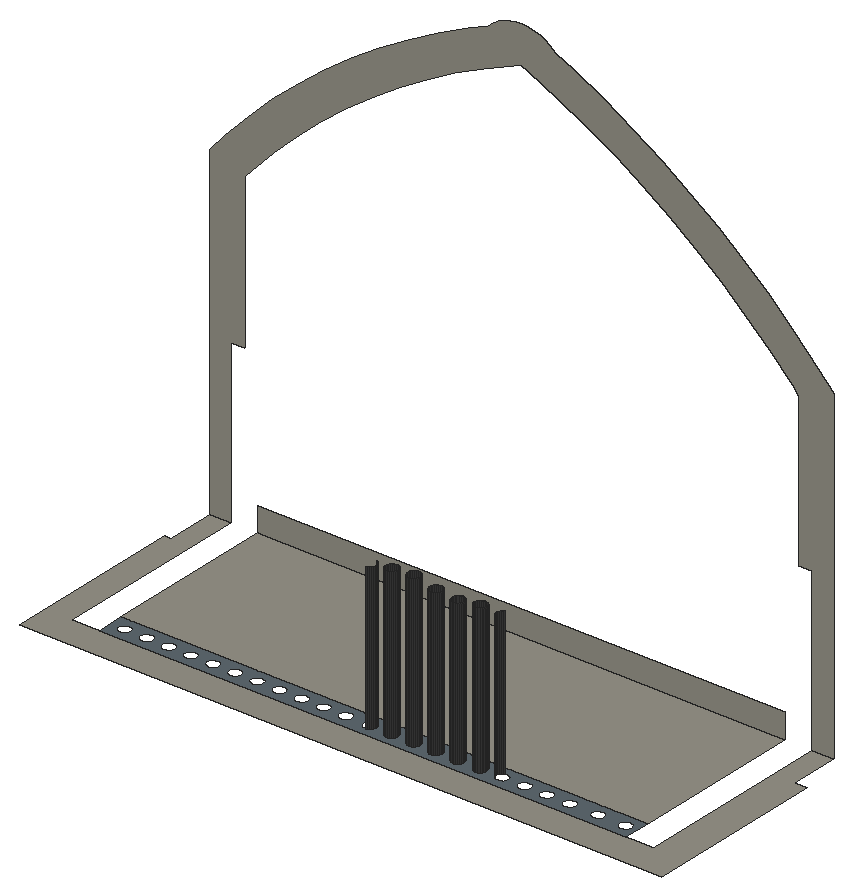
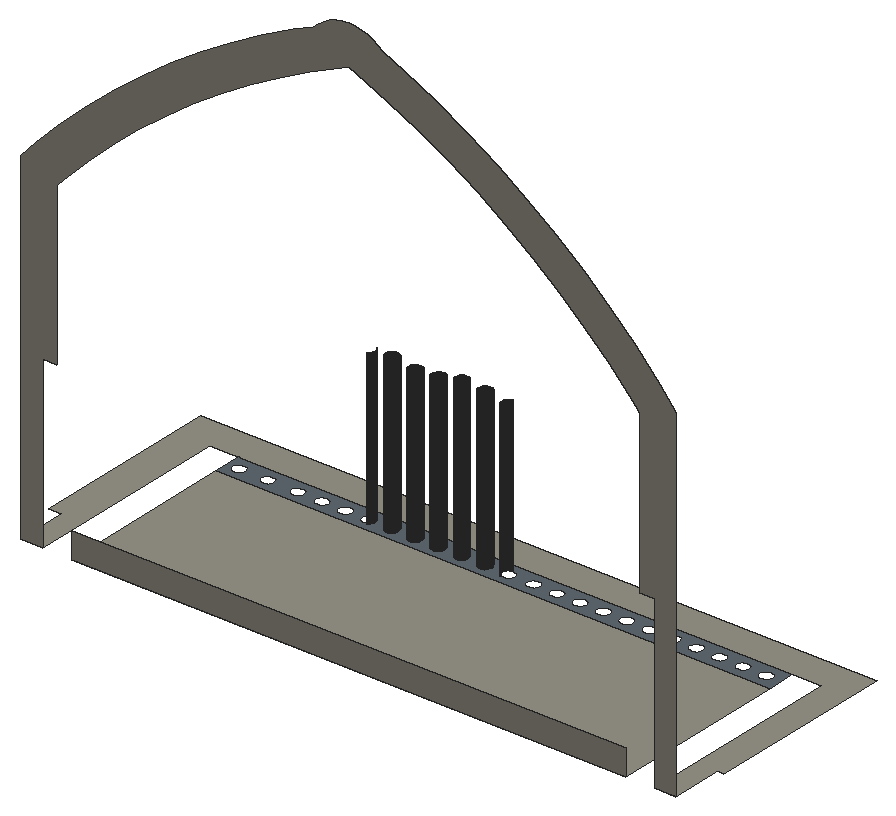
# SketchUp Ruby script. Lengths in inches.
U = 1.inch
M = Sketchup.active_model
def pt(a) = Geom::Point3d.new(a.map { |v| v * U })
def face(e, loops, mat)
  f = e.add_face(loops[0].map { |a| pt(a) })
  loops[1..].each { |l| e.add_face(l.map { |a| pt(a) }).erase! }
  f.material = f.back_material = mat if mat
  f
end
# faces: each face lists its corners as indices into pts; further lists are holes
def faces(e, pts, list, mat = nil) = list.each { |f| face(e, (f[0].is_a?(Array) ? f : [f]).map { |l| l.map { |i| pts[i] } }, mat) }
# xy, xz, yz: faces in a plane at the given z, y or x. An outline is a flat list of corners, or four numbers for a rectangle; further outlines are holes
def ring(l) = l.size == 4 ? [[l[0], l[1]], [l[2], l[1]], [l[2], l[3]], [l[0], l[3]]] : l.each_slice(2).to_a
def flat(e, list, mat, &to3) = list.each { |f| face(e, (f[0].is_a?(Array) ? f : [f]).map { |l| ring(l).map { |u, v| to3.(u, v) } }, mat) }
def xy(e, z, list, mat = nil) = flat(e, list, mat) { |x, y| [x, y, z] }
def xz(e, y, list, mat = nil) = flat(e, list, mat) { |x, z| [x, y, z] }
def yz(e, x, list, mat = nil) = flat(e, list, mat) { |y, z| [x, y, z] }
def lines(e, pts, list) = list.each { |a, b| e.add_line(pt(pts[a]), pt(pts[b])) }
# prism: a flat outline (further loops are holes) pulled along v
def prism(e, loops, v, mat = nil)
  f = face(e, loops, mat); d = Geom::Vector3d.new(v.map { |x| x * U })
  f.pushpull(f.normal.samedirection?(d) ? d.length : -d.length)
end
def box(e, o, s, mat = nil) = prism(e, [[o, [o[0] + s[0], o[1], o[2]], [o[0] + s[0], o[1] + s[1], o[2]], [o[0], o[1] + s[1], o[2]]]], [0, 0, s[2]], mat)
def at(x, y, z, deg = 0) = Geom::Transformation.translation(pt([x, y, z])) * Geom::Transformation.rotation(ORIGIN, Z_AXIS, deg.degrees)
def axes(o, x, y, z) = Geom::Transformation.new([*x, 0, *y, 0, *z, 0, *pt(o).to_a, 1])
def part(name) = M.definitions.add(name)
# library, detail: a bought-in or finely detailed component or shape, given as its bounding box
def library(name, o, s) = part(name).tap { |d| box(d.entities, o, s) }
def detail(e, o, s) = box(e.add_group.entities, o, s)
def put(e, d, t, mat = nil) = e.add_instance(d, t).tap { |i| i.material = mat if mat }
def group(e, t, mat = nil) = e.add_group.tap { |g| g.transformation = t; g.material = mat if mat }.entities
root = M.entities
M.materials.add("[Color M07]").color = [58, 58, 58]
M.materials.add("[Formica Graystone]").color = [149, 146, 135]
M.materials.add("[Formica Speckled Grey]").color = [94, 105, 111]
xy(root,452.9,[[260.4,119.22,260.2,119.27,260.01,119.375,259.86,119.52,259.75,119.71,259.69,119.91,259.69,120.125,259.75,120.33,259.85,120.51,260,120.67,260.18,120.77,260.38,120.83,260.6,120.83,260.8,120.78,260.99,120.68,261.14,120.53,261.25,120.35,261.3,120.14,261.31,119.93,261.25,119.72,261.15,119.54,261,119.39,260.82,119.28,260.61,119.22],[263.28,119.22,263.07,119.27,262.89,119.375,262.73,119.52,262.625,119.71,262.57,119.91,262.57,120.125,262.62,120.33,262.72,120.51,262.87,120.67,263.05,120.77,263.26,120.83,263.47,120.83,263.68,120.78,263.86,120.68,264.01,120.53,264.12,120.35,264.18,120.14,264.18,119.93,264.13,119.72,264.02,119.54,263.875,119.39,263.69,119.28,263.49,119.22],[266.15,119.22,265.95,119.27,265.76,119.375,265.61,119.52,265.5,119.71,265.44,119.91,265.44,120.125,265.5,120.33,265.6,120.51,265.75,120.67,265.93,120.77,266.13,120.83,266.35,120.83,266.55,120.78,266.74,120.68,266.89,120.53,267,120.35,267.05,120.14,267.06,119.93,267,119.72,266.9,119.54,266.75,119.39,266.57,119.28,266.36,119.22],[269.03,119.22,268.82,119.27,268.64,119.375,268.48,119.52,268.375,119.71,268.32,119.91,268.32,120.125,268.37,120.33,268.47,120.51,268.62,120.67,268.8,120.77,269.01,120.83,269.22,120.83,269.43,120.78,269.61,120.68,269.76,120.53,269.87,120.35,269.93,120.14,269.93,119.93,269.88,119.72,269.77,119.54,269.625,119.39,269.44,119.28,269.24,119.22],[271.9,119.22,271.7,119.27,271.51,119.375,271.36,119.52,271.25,119.71,271.19,119.91,271.19,120.125,271.25,120.33,271.35,120.51,271.5,120.67,271.68,120.77,271.88,120.83,272.1,120.83,272.3,120.78,272.49,120.68,272.64,120.53,272.75,120.35,272.8,120.14,272.81,119.93,272.75,119.72,272.65,119.54,272.5,119.39,272.32,119.28,272.11,119.22]])
xy(root,452.9,[[216.84,114.16,300.34,114.16,300.34,137.66,298.71,137.66,298.71,144.04,295.93,144.04,295.93,118.22,220.36,118.22,220.36,144.04,217.65,144.04,217.65,137.66,216.84,137.66],[223.91,121.78,292.38,144.04]],"[Formica Graystone]")
xy(root,452.9,[[[223.91,118.22,292.38,121.78],[225.65,119.22,225.45,119.27,225.26,119.375,225.11,119.52,225,119.71,224.94,119.91,224.94,120.125,225,120.33,225.1,120.51,225.25,120.67,225.43,120.77,225.63,120.83,225.85,120.83,226.05,120.78,226.24,120.68,226.39,120.53,226.5,120.35,226.55,120.14,226.56,119.93,226.5,119.72,226.4,119.54,226.25,119.39,226.07,119.28,225.86,119.22],[228.53,119.22,228.32,119.27,228.14,119.375,227.98,119.52,227.875,119.71,227.82,119.91,227.82,120.125,227.87,120.33,227.97,120.51,228.12,120.67,228.3,120.77,228.51,120.83,228.72,120.83,228.93,120.78,229.11,120.68,229.26,120.53,229.37,120.35,229.43,120.14,229.43,119.93,229.38,119.72,229.27,119.54,229.125,119.39,228.94,119.28,228.74,119.22],[231.4,119.22,231.2,119.27,231.01,119.375,230.86,119.52,230.75,119.71,230.69,119.91,230.69,120.125,230.75,120.33,230.85,120.51,231,120.67,231.18,120.77,231.38,120.83,231.6,120.83,231.8,120.78,231.99,120.68,232.14,120.53,232.25,120.35,232.3,120.14,232.31,119.93,232.25,119.72,232.15,119.54,232,119.39,231.82,119.28,231.61,119.22],[234.28,119.22,234.07,119.27,233.89,119.375,233.73,119.52,233.625,119.71,233.57,119.91,233.57,120.125,233.62,120.33,233.72,120.51,233.87,120.67,234.05,120.77,234.26,120.83,234.47,120.83,234.68,120.78,234.86,120.68,235.01,120.53,235.12,120.35,235.18,120.14,235.18,119.93,235.13,119.72,235.02,119.54,234.875,119.39,234.69,119.28,234.49,119.22],[237.15,119.22,236.95,119.27,236.76,119.375,236.61,119.52,236.5,119.71,236.44,119.91,236.44,120.125,236.5,120.33,236.6,120.51,236.75,120.67,236.93,120.77,237.13,120.83,237.35,120.83,237.55,120.78,237.74,120.68,237.89,120.53,238,120.35,238.05,120.14,238.06,119.93,238,119.72,237.9,119.54,237.75,119.39,237.57,119.28,237.36,119.22],[240.03,119.22,239.82,119.27,239.64,119.375,239.48,119.52,239.375,119.71,239.32,119.91,239.32,120.125,239.37,120.33,239.47,120.51,239.62,120.67,239.8,120.77,240.01,120.83,240.22,120.83,240.43,120.78,240.61,120.68,240.76,120.53,240.87,120.35,240.93,120.14,240.93,119.93,240.88,119.72,240.77,119.54,240.625,119.39,240.44,119.28,240.24,119.22],[242.9,119.22,242.7,119.27,242.51,119.375,242.36,119.52,242.25,119.71,242.19,119.91,242.19,120.125,242.25,120.33,242.35,120.51,242.5,120.67,242.68,120.77,242.88,120.83,243.1,120.83,243.3,120.78,243.49,120.68,243.64,120.53,243.75,120.35,243.8,120.14,243.81,119.93,243.75,119.72,243.65,119.54,243.5,119.39,243.32,119.28,243.11,119.22],[245.78,119.22,245.57,119.27,245.39,119.375,245.23,119.52,245.125,119.71,245.07,119.91,245.07,120.125,245.12,120.33,245.22,120.51,245.37,120.67,245.55,120.77,245.76,120.83,245.97,120.83,246.18,120.78,246.36,120.68,246.51,120.53,246.62,120.35,246.68,120.14,246.68,119.93,246.63,119.72,246.52,119.54,246.375,119.39,246.19,119.28,245.99,119.22],[248.65,119.22,248.45,119.27,248.26,119.375,248.11,119.52,248,119.71,247.94,119.91,247.94,120.125,248,120.33,248.1,120.51,248.25,120.67,248.43,120.77,248.63,120.83,248.85,120.83,249.05,120.78,249.24,120.68,249.39,120.53,249.5,120.35,249.55,120.14,249.56,119.93,249.5,119.72,249.4,119.54,249.25,119.39,249.07,119.28,248.86,119.22],[251.53,119.22,251.32,119.27,251.14,119.375,250.98,119.52,250.875,119.71,250.82,119.91,250.82,120.125,250.87,120.33,250.97,120.51,251.12,120.67,251.3,120.77,251.51,120.83,251.72,120.83,251.93,120.78,252.11,120.68,252.26,120.53,252.37,120.35,252.43,120.14,252.43,119.93,252.38,119.72,252.27,119.54,252.125,119.39,251.94,119.28,251.74,119.22],[254.4,119.22,254.2,119.27,254.01,119.375,253.86,119.52,253.75,119.71,253.69,119.91,253.69,120.125,253.75,120.33,253.85,120.51,254,120.67,254.18,120.77,254.38,120.83,254.6,120.83,254.8,120.78,254.99,120.68,255.14,120.53,255.25,120.35,255.3,120.14,255.31,119.93,255.25,119.72,255.15,119.54,255,119.39,254.82,119.28,254.61,119.22],[257.53,119.22,257.32,119.27,257.14,119.375,256.98,119.52,256.875,119.71,256.82,119.91,256.82,120.125,256.87,120.33,256.97,120.51,257.12,120.67,257.3,120.77,257.51,120.83,257.72,120.83,257.93,120.78,258.11,120.68,258.26,120.53,258.37,120.35,258.43,120.14,258.43,119.93,258.38,119.72,258.27,119.54,258.125,119.39,257.94,119.28,257.74,119.22],[260.4,119.22,260.2,119.27,260.01,119.375,259.86,119.52,259.75,119.71,259.69,119.91,259.69,120.125,259.75,120.33,259.85,120.51,260,120.67,260.18,120.77,260.38,120.83,260.6,120.83,260.8,120.78,260.99,120.68,261.14,120.53,261.25,120.35,261.3,120.14,261.31,119.93,261.25,119.72,261.15,119.54,261,119.39,260.82,119.28,260.61,119.22],[263.28,119.22,263.07,119.27,262.89,119.375,262.73,119.52,262.625,119.71,262.57,119.91,262.57,120.125,262.62,120.33,262.72,120.51,262.87,120.67,263.05,120.77,263.26,120.83,263.47,120.83,263.68,120.78,263.86,120.68,264.01,120.53,264.12,120.35,264.18,120.14,264.18,119.93,264.13,119.72,264.02,119.54,263.875,119.39,263.69,119.28,263.49,119.22],[266.15,119.22,265.95,119.27,265.76,119.375,265.61,119.52,265.5,119.71,265.44,119.91,265.44,120.125,265.5,120.33,265.6,120.51,265.75,120.67,265.93,120.77,266.13,120.83,266.35,120.83,266.55,120.78,266.74,120.68,266.89,120.53,267,120.35,267.05,120.14,267.06,119.93,267,119.72,266.9,119.54,266.75,119.39,266.57,119.28,266.36,119.22],[269.03,119.22,268.82,119.27,268.64,119.375,268.48,119.52,268.375,119.71,268.32,119.91,268.32,120.125,268.37,120.33,268.47,120.51,268.62,120.67,268.8,120.77,269.01,120.83,269.22,120.83,269.43,120.78,269.61,120.68,269.76,120.53,269.87,120.35,269.93,120.14,269.93,119.93,269.88,119.72,269.77,119.54,269.625,119.39,269.44,119.28,269.24,119.22],[271.9,119.22,271.7,119.27,271.51,119.375,271.36,119.52,271.25,119.71,271.19,119.91,271.19,120.125,271.25,120.33,271.35,120.51,271.5,120.67,271.68,120.77,271.88,120.83,272.1,120.83,272.3,120.78,272.49,120.68,272.64,120.53,272.75,120.35,272.8,120.14,272.81,119.93,272.75,119.72,272.65,119.54,272.5,119.39,272.32,119.28,272.11,119.22],[274.78,119.22,274.57,119.27,274.39,119.375,274.23,119.52,274.125,119.71,274.07,119.91,274.07,120.125,274.12,120.33,274.22,120.51,274.37,120.67,274.55,120.77,274.76,120.83,274.97,120.83,275.18,120.78,275.36,120.68,275.51,120.53,275.62,120.35,275.68,120.14,275.68,119.93,275.63,119.72,275.52,119.54,275.375,119.39,275.19,119.28,274.99,119.22],[277.65,119.22,277.45,119.27,277.26,119.375,277.11,119.52,277,119.71,276.94,119.91,276.94,120.125,277,120.33,277.1,120.51,277.25,120.67,277.43,120.77,277.63,120.83,277.85,120.83,278.05,120.78,278.24,120.68,278.39,120.53,278.5,120.35,278.55,120.14,278.56,119.93,278.5,119.72,278.4,119.54,278.25,119.39,278.07,119.28,277.86,119.22],[280.53,119.22,280.32,119.27,280.14,119.375,279.98,119.52,279.875,119.71,279.82,119.91,279.82,120.125,279.87,120.33,279.97,120.51,280.12,120.67,280.3,120.77,280.51,120.83,280.72,120.83,280.93,120.78,281.11,120.68,281.26,120.53,281.37,120.35,281.43,120.14,281.43,119.93,281.38,119.72,281.27,119.54,281.125,119.39,280.94,119.28,280.74,119.22],[290.78,119.22,290.57,119.27,290.39,119.375,290.23,119.52,290.125,119.71,290.07,119.91,290.07,120.125,290.12,120.33,290.22,120.51,290.37,120.67,290.55,120.77,290.76,120.83,290.97,120.83,291.18,120.78,291.36,120.68,291.51,120.53,291.62,120.35,291.68,120.14,291.68,119.93,291.63,119.72,291.52,119.54,291.375,119.39,291.19,119.28,290.99,119.22],[283.53,119.22,283.32,119.27,283.14,119.375,282.98,119.52,282.875,119.71,282.82,119.91,282.82,120.125,282.87,120.33,282.97,120.51,283.12,120.67,283.3,120.77,283.51,120.83,283.72,120.83,283.93,120.78,284.11,120.68,284.26,120.53,284.37,120.35,284.43,120.14,284.43,119.93,284.38,119.72,284.27,119.54,284.125,119.39,283.94,119.28,283.74,119.22],[287.21,119.22,287.01,119.27,286.82,119.375,286.67,119.52,286.5625,119.71,286.51,119.91,286.5,120.125,286.56,120.33,286.66,120.51,286.81,120.67,286.99,120.77,287.2,120.83,287.41,120.83,287.61,120.78,287.8,120.68,287.95,120.53,288.06,120.35,288.12,120.14,288.12,119.93,288.07,119.72,287.96,119.54,287.8125,119.39,287.63,119.28,287.43,119.22]]],"[Formica Speckled Grey]")
xz(root,119.22,[[260.4,452.9,260.61,472.27],[263.28,452.9,263.49,472.48],[266.15,452.9,266.36,471.82],[269.03,452.9,269.24,471.61],[271.9,452.9,272.11,472.05]],"[Color M07]")
xz(root,120.83,[[260.38,452.9,260.6,472.27],[263.26,452.9,263.47,472.48],[266.13,452.9,266.35,471.82],[269.01,452.9,269.22,471.61],[271.88,452.9,272.1,472.05]],"[Color M07]")
xz(root,144.04,[[217.65,452.9,220.36,452.9,220.36,473.83,222.16,473.83,222.16,493.75,223.04,494.78,225.91,497.87,228.92,500.82,232.06,503.64,235.32,506.31,238.7,508.83,242.1875,511.2,245.78,513.41,249.47,515.46,253.24,517.33,257.1,519.04,258.07,519.42,259.04,519.01,262.89,517.22,266.65,515.27,270.34,513.16,273.94,510.92,277.45,508.52,280.85,505.99,284.15,503.33,287.34,500.53,290.42,497.6,293.375,494.56,294.2,493.63,294.2,473.83,295.93,473.83,295.93,452.9,298.71,452.9,298.71,495.36,296.67,497.63,293.59,500.81,290.38,503.86,287.06,506.78,283.61,509.56,280.0625,512.2,276.41,514.69,272.65,517.04,268.81,519.23,264.88,521.26,262.4,522.42,261.83,522.96,261.18,523.41,260.48,523.78,259.74,524.05,258.97,524.22,258.1875,524.29,258.14,524.28,258.12,524.28,257.4,524.25,256.62,524.1,255.87,523.86,255.16,523.51,254.5,523.08,253.91,522.5625,251.32,521.42,247.37,519.45,243.5,517.3,239.74,514.99,236.08,512.5,232.54,509.86,229.125,507.06,225.83,504.11,222.68,501.01,219.67,497.78,217.65,495.41],[223.91,452.9,292.38,456.09]],"[Formica Graystone]")
yz(root,258.43,[[119.93,452.9,120.14,471.82]],"[Color M07]")
yz(root,259.69,[[119.91,452.9,120.125,472.27]],"[Color M07]")
yz(root,262.57,[[119.91,452.9,120.125,472.48]],"[Color M07]")
yz(root,264.18,[[119.93,452.9,120.14,472.48]],"[Color M07]")
yz(root,265.44,[[119.91,452.9,120.125,471.82]],"[Color M07]")
yz(root,268.32,[[119.91,452.9,120.125,471.61]],"[Color M07]")
yz(root,269.93,[[119.93,452.9,120.14,471.61]],"[Color M07]")
yz(root,271.19,[[119.91,452.9,120.125,472.05]],"[Color M07]")
yz(root,274.07,[[119.91,452.9,120.125,471.83]],"[Color M07]")
p = [[257.74,119.22,452.9],[257.94,119.28,452.9],[257.94,119.28,471.82],[257.74,119.22,471.82],[260.2,119.27,452.9],[260.4,119.22,452.9],
  [260.4,119.22,472.27],[260.2,119.27,472.27],[260.61,119.22,452.9],[260.82,119.28,452.9],[260.82,119.28,472.27],[260.61,119.22,472.27],
  [263.07,119.27,452.9],[263.28,119.22,452.9],[263.28,119.22,472.48],[263.07,119.27,472.48],[263.49,119.22,452.9],[263.69,119.28,452.9],
  [263.69,119.28,472.48],[263.49,119.22,472.48],[265.95,119.27,452.9],[266.15,119.22,452.9],[266.15,119.22,471.82],[265.95,119.27,471.82],
  [266.36,119.22,452.9],[266.57,119.28,452.9],[266.57,119.28,471.82],[266.36,119.22,471.82],[268.82,119.27,452.9],[269.03,119.22,452.9],
  [269.03,119.22,471.61],[268.82,119.27,471.61],[269.24,119.22,452.9],[269.44,119.28,452.9],[269.44,119.28,471.61],[269.24,119.22,471.61],
  [271.7,119.27,452.9],[271.9,119.22,452.9],[271.9,119.22,472.05],[271.7,119.27,472.05],[272.11,119.22,452.9],[272.32,119.28,452.9],
  [272.32,119.28,472.05],[272.11,119.22,472.05],[258.125,119.39,452.9],[258.125,119.39,471.82],[260.01,119.375,452.9],[260.01,119.375,472.27],
  [261,119.39,452.9],[261,119.39,472.27],[262.89,119.375,452.9],[262.89,119.375,472.48],[263.875,119.39,452.9],[263.875,119.39,472.48],
  [265.76,119.375,452.9],[265.76,119.375,471.82],[266.75,119.39,452.9],[266.75,119.39,471.82],[268.64,119.375,452.9],[268.64,119.375,471.61],
  [269.625,119.39,452.9],[269.625,119.39,471.61],[271.51,119.375,452.9],[271.51,119.375,472.05],[272.5,119.39,452.9],[272.5,119.39,472.05],
  [258.27,119.54,452.9],[258.27,119.54,471.82],[259.86,119.52,452.9],[259.86,119.52,472.27],[261.15,119.54,452.9],[261.15,119.54,472.27],
  [262.73,119.52,452.9],[262.73,119.52,472.48],[264.02,119.54,452.9],[264.02,119.54,472.48],[265.61,119.52,452.9],[265.61,119.52,471.82],
  [266.9,119.54,452.9],[266.9,119.54,471.82],[268.48,119.52,452.9],[268.48,119.52,471.61],[269.77,119.54,452.9],[269.77,119.54,471.61],
  [271.36,119.52,452.9],[271.36,119.52,472.05],[272.65,119.54,452.9],[272.65,119.54,472.05],[274.23,119.52,452.9],[274.39,119.375,452.9],
  [274.39,119.375,471.83],[274.23,119.52,471.83],[258.38,119.72,452.9],[258.38,119.72,471.82],[259.75,119.71,452.9],[259.75,119.71,472.27],
  [261.25,119.72,452.9],[261.25,119.72,472.27],[262.625,119.71,452.9],[262.625,119.71,472.48],[264.13,119.72,452.9],[264.13,119.72,472.48],
  [265.5,119.71,452.9],[265.5,119.71,471.82],[267,119.72,452.9],[267,119.72,471.82],[268.375,119.71,452.9],[268.375,119.71,471.61],
  [269.88,119.72,452.9],[269.88,119.72,471.61],[271.25,119.71,452.9],[271.25,119.71,472.05],[272.75,119.72,452.9],[272.75,119.72,472.05],
  [274.125,119.71,452.9],[274.125,119.71,471.83],[258.43,119.93,452.9],[258.43,119.93,471.82],[259.69,119.91,452.9],[259.69,119.91,472.27],
  [261.31,119.93,452.9],[261.31,119.93,472.27],[262.57,119.91,452.9],[262.57,119.91,472.48],[264.18,119.93,452.9],[264.18,119.93,472.48],
  [265.44,119.91,452.9],[265.44,119.91,471.82],[267.06,119.93,452.9],[267.06,119.93,471.82],[268.32,119.91,452.9],[268.32,119.91,471.61],
  [269.93,119.93,452.9],[269.93,119.93,471.61],[271.19,119.91,452.9],[271.19,119.91,472.05],[272.81,119.93,452.9],[272.81,119.93,472.05],
  [274.07,119.91,452.9],[274.07,119.91,471.83],[261.3,120.14,452.9],[261.3,120.14,472.27],[267.05,120.14,452.9],[267.05,120.14,471.82],
  [272.8,120.14,452.9],[272.8,120.14,472.05],[258.43,120.14,452.9],[258.37,120.35,452.9],[258.37,120.35,471.82],[258.43,120.14,471.82],
  [259.75,120.33,452.9],[259.69,120.125,452.9],[259.69,120.125,472.27],[259.75,120.33,472.27],[261.25,120.35,452.9],[261.25,120.35,472.27],
  [262.62,120.33,452.9],[262.57,120.125,452.9],[262.57,120.125,472.48],[262.62,120.33,472.48],[264.18,120.14,452.9],[264.12,120.35,452.9],
  [264.12,120.35,472.48],[264.18,120.14,472.48],[265.5,120.33,452.9],[265.44,120.125,452.9],[265.44,120.125,471.82],[265.5,120.33,471.82],
  [267,120.35,452.9],[267,120.35,471.82],[268.37,120.33,452.9],[268.32,120.125,452.9],[268.32,120.125,471.61],[268.37,120.33,471.61],
  [269.93,120.14,452.9],[269.87,120.35,452.9],[269.87,120.35,471.61],[269.93,120.14,471.61],[271.25,120.33,452.9],[271.19,120.125,452.9],
  [271.19,120.125,472.05],[271.25,120.33,472.05],[272.75,120.35,452.9],[272.75,120.35,472.05],[274.12,120.33,452.9],[274.07,120.125,452.9],
  [274.07,120.125,471.83],[274.12,120.33,471.83],[258.26,120.53,452.9],[258.26,120.53,471.82],[259.85,120.51,452.9],[259.85,120.51,472.27],
  [261.14,120.53,452.9],[261.14,120.53,472.27],[262.72,120.51,452.9],[262.72,120.51,472.48],[264.01,120.53,452.9],[264.01,120.53,472.48],
  [265.6,120.51,452.9],[265.6,120.51,471.82],[266.89,120.53,452.9],[266.89,120.53,471.82],[268.47,120.51,452.9],[268.47,120.51,471.61],
  [269.76,120.53,452.9],[269.76,120.53,471.61],[271.35,120.51,452.9],[271.35,120.51,472.05],[272.64,120.53,452.9],[272.64,120.53,472.05],
  [274.22,120.51,452.9],[274.22,120.51,471.83],[258.11,120.68,452.9],[258.11,120.68,471.82],[260,120.67,452.9],[260,120.67,472.27],
  [260.99,120.68,452.9],[260.99,120.68,472.27],[262.87,120.67,452.9],[262.83,120.62,472.48],[262.87,120.67,472.48],[263.86,120.68,452.9],
  [263.86,120.68,472.48],[263.92,120.62,472.48],[265.75,120.67,452.9],[265.75,120.67,471.82],[266.74,120.68,452.9],[266.74,120.68,471.82],
  [268.62,120.67,452.9],[268.58,120.62,471.61],[268.62,120.67,471.61],[269.61,120.68,452.9],[269.61,120.68,471.61],[269.67,120.62,471.61],
  [271.5,120.67,452.9],[271.5,120.67,472.05],[272.49,120.68,452.9],[272.49,120.68,472.05],[274.37,120.67,452.9],[274.37,120.67,471.83],
  [257.93,120.78,452.9],[257.93,120.78,471.82],[258.06,120.71,471.82],[260.18,120.77,452.9],[260.07,120.71,472.27],[260.18,120.77,472.27],
  [260.8,120.78,452.9],[260.8,120.78,472.27],[260.93,120.71,472.27],[263.05,120.77,452.9],[263.05,120.77,472.48],[263.68,120.78,452.9],
  [263.68,120.78,472.48],[265.93,120.77,452.9],[265.82,120.71,471.82],[265.93,120.77,471.82],[266.55,120.78,452.9],[266.55,120.78,471.82],
  [266.68,120.71,471.82],[268.8,120.77,452.9],[268.8,120.77,471.61],[269.43,120.78,452.9],[269.43,120.78,471.61],[271.68,120.77,452.9],
  [271.62,120.74,472.05],[271.68,120.77,472.05],[272.3,120.78,452.9],[272.3,120.78,472.05],[272.38,120.74,472.05],[274.55,120.77,452.9],
  [274.55,120.77,471.83],[260.38,120.83,452.9],[260.38,120.83,472.27],[260.6,120.83,452.9],[260.6,120.83,472.27],[263.26,120.83,452.9],
  [263.26,120.83,472.48],[263.47,120.83,452.9],[263.47,120.83,472.48],[266.13,120.83,452.9],[266.13,120.83,471.82],[266.35,120.83,452.9],
  [266.35,120.83,471.82],[269.01,120.83,452.9],[269.01,120.83,471.61],[269.22,120.83,452.9],[269.22,120.83,471.61],[271.88,120.83,452.9],
  [271.88,120.83,472.05],[272.1,120.83,452.9],[272.1,120.83,472.05]]
faces(root,p,[[0,1,2,3],[4,5,6,7],[8,9,10,11],[12,13,14,15],[16,17,18,19],[20,21,22,23],[24,25,26,27],[28,29,30,31],
  [32,33,34,35],[36,37,38,39],[40,41,42,43],[1,44,45,2],[46,4,7,47],[9,48,49,10],[50,12,15,51],[17,52,53,18],
  [54,20,23,55],[25,56,57,26],[58,28,31,59],[33,60,61,34],[62,36,39,63],[41,64,65,42],[44,66,67,45],[68,46,47,69],
  [48,70,71,49],[72,50,51,73],[52,74,75,53],[76,54,55,77],[56,78,79,57],[80,58,59,81],[60,82,83,61],[84,62,63,85],
  [64,86,87,65],[88,89,90,91],[66,92,93,67],[94,68,69,95],[70,96,97,71],[98,72,73,99],[74,100,101,75],[102,76,77,103],
  [78,104,105,79],[106,80,81,107],[82,108,109,83],[110,84,85,111],[86,112,113,87],[114,88,91,115],[92,116,117,93],[118,94,95,119],
  [96,120,121,97],[122,98,99,123],[100,124,125,101],[126,102,103,127],[104,128,129,105],[130,106,107,131],[108,132,133,109],[134,110,111,135],
  [112,136,137,113],[138,114,115,139],[120,140,141,121],[128,142,143,129],[136,144,145,137],[146,147,148,149],[150,151,152,153],[140,154,155,141],
  [156,157,158,159],[160,161,162,163],[164,165,166,167],[142,168,169,143],[170,171,172,173],[174,175,176,177],[178,179,180,181],[144,182,183,145],
  [184,185,186,187],[147,188,189,148],[190,150,153,191],[154,192,193,155],[194,156,159,195],[161,196,197,162],[198,164,167,199],[168,200,201,169],
  [202,170,173,203],[175,204,205,176],[206,178,181,207],[182,208,209,183],[210,184,187,211],[188,212,213,189],[214,190,191,215],[192,216,217,193],
  [218,194,195,219,220],[196,221,222,223,197],[224,198,199,225],[200,226,227,201],[228,202,203,229,230],[204,231,232,233,205],[234,206,207,235],[208,236,237,209],
  [238,210,211,239],[212,240,241,242,213],[243,214,215,244,245],[216,246,247,248,217],[249,218,220,250],[221,251,252,222],[253,224,225,254,255],[226,256,257,258,227],
  [259,228,230,260],[231,261,262,232],[263,234,235,264,265],[236,266,267,268,237],[269,238,239,270],[271,243,245,272],[246,273,274,247],[275,249,250,276],
  [251,277,278,252],[279,253,255,280],[256,281,282,257],[283,259,260,284],[261,285,286,262],[287,263,265,288],[266,289,290,267]],"[Color M07]")
